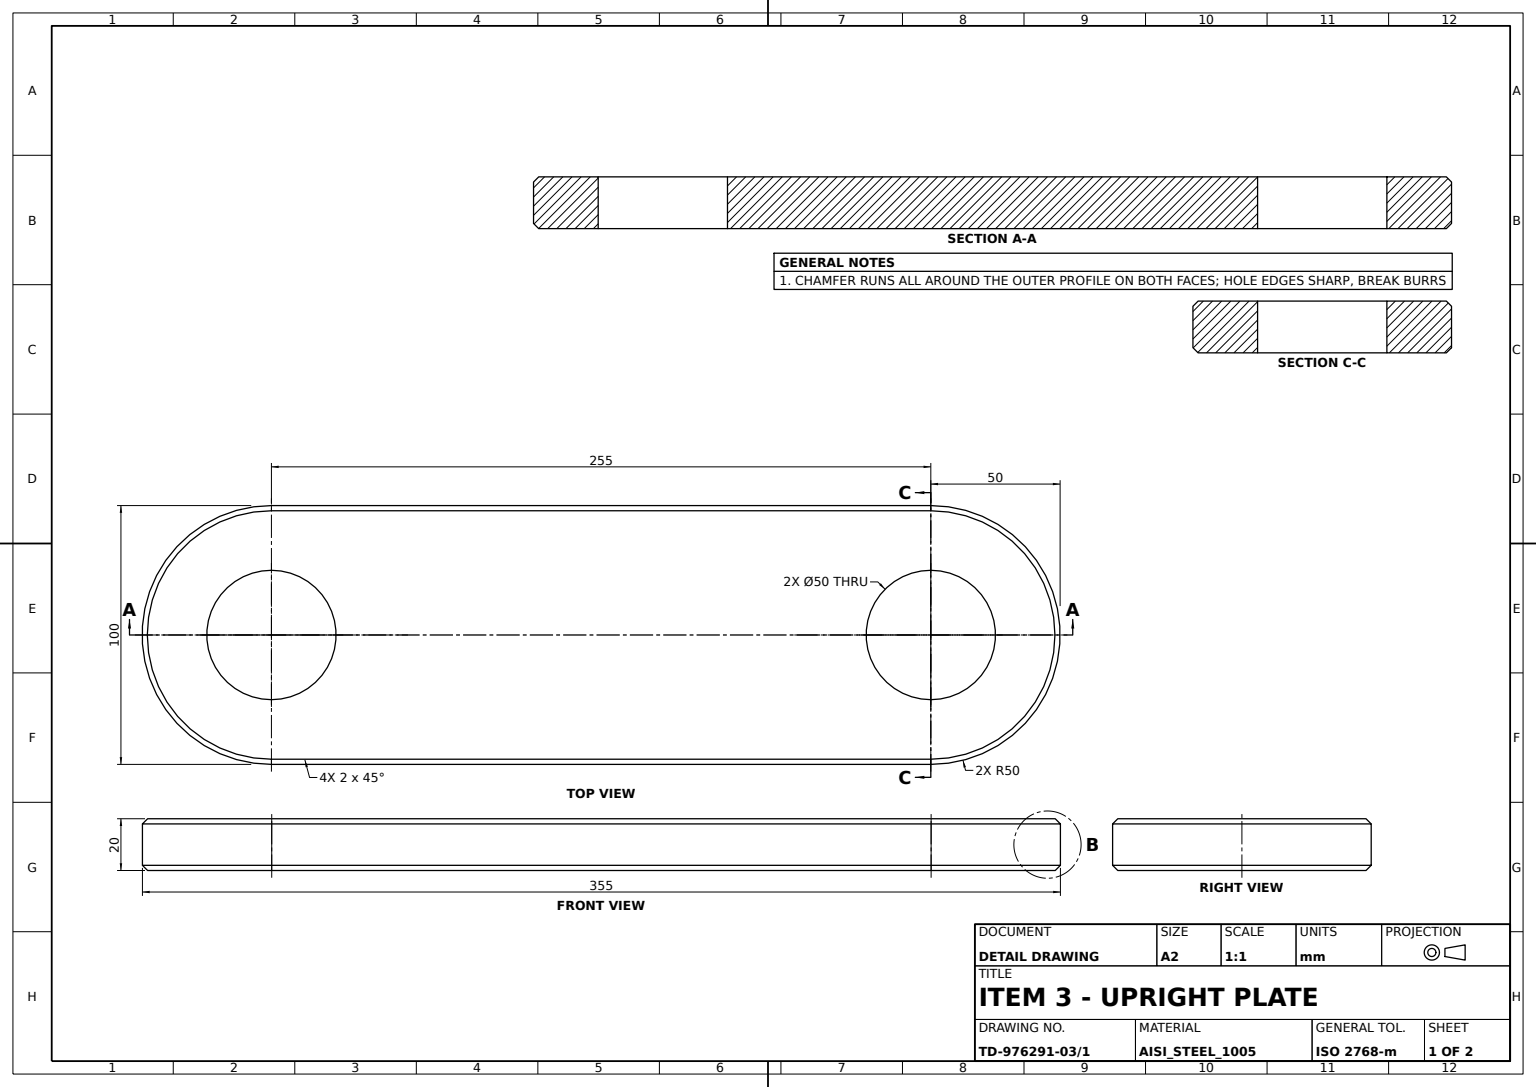
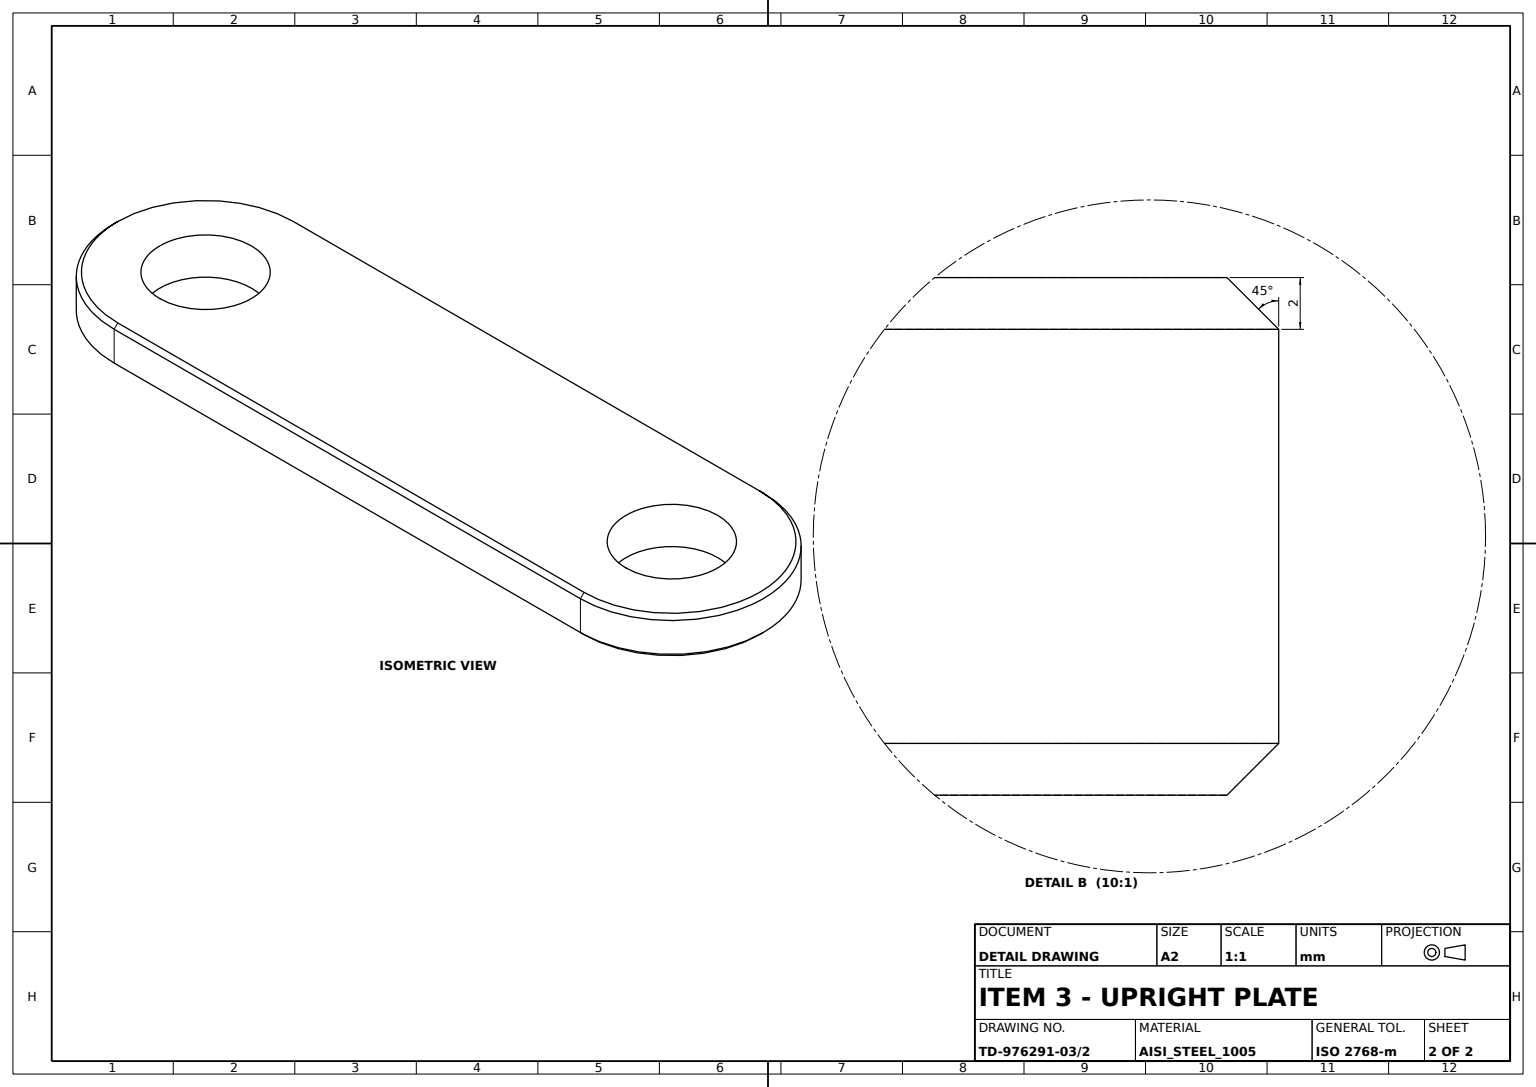
ISO-10303-21;
HEADER;
FILE_DESCRIPTION((''),'2;1');
FILE_NAME('','',(''),(''),'','','');
FILE_SCHEMA(('AUTOMOTIVE_DESIGN'));
ENDSEC;
DATA;
#1=APPLICATION_CONTEXT('');
#2=PRODUCT_CONTEXT('',#1,'mechanical');
#3=PRODUCT('','','',(#2));
#4=PRODUCT_DEFINITION_FORMATION('','',#3);
#5=PRODUCT_DEFINITION_CONTEXT('',#1,'design');
#6=PRODUCT_DEFINITION('','',#4,#5);
#7=PRODUCT_DEFINITION_SHAPE('','',#6);
#8=(LENGTH_UNIT()NAMED_UNIT(*)SI_UNIT(.MILLI.,.METRE.));
#9=(NAMED_UNIT(*)PLANE_ANGLE_UNIT()SI_UNIT($,.RADIAN.));
#10=(NAMED_UNIT(*)SI_UNIT($,.STERADIAN.)SOLID_ANGLE_UNIT());
#11=UNCERTAINTY_MEASURE_WITH_UNIT(LENGTH_MEASURE(0.005),#8,'distance_accuracy_value','');
#12=(GEOMETRIC_REPRESENTATION_CONTEXT(3)GLOBAL_UNCERTAINTY_ASSIGNED_CONTEXT((#11))GLOBAL_UNIT_ASSIGNED_CONTEXT((#8,#9,#10))REPRESENTATION_CONTEXT('',''));
#13=CARTESIAN_POINT('',(-50.,-2.,127.5));
#14=VERTEX_POINT('',#13);
#15=CARTESIAN_POINT('',(-48.,0.,127.5));
#16=VERTEX_POINT('',#15);
#17=DIRECTION('',(0.707106781,0.707106781,0.));
#18=VECTOR('',#17,1000.);
#19=LINE('',#13,#18);
#20=EDGE_CURVE('',#14,#16,#19,.T.);
#21=ORIENTED_EDGE('',*,*,#20,.F.);
#22=CARTESIAN_POINT('',(50.,-2.,127.5));
#23=VERTEX_POINT('',#22);
#24=CARTESIAN_POINT('',(0.,-2.,127.5));
#25=DIRECTION('',(0.,-1.,0.));
#26=DIRECTION('',(0.,0.,-1.));
#27=AXIS2_PLACEMENT_3D('',#24,#25,#26);
#28=CIRCLE('',#27,50.);
#29=EDGE_CURVE('',#23,#14,#28,.T.);
#30=ORIENTED_EDGE('',*,*,#29,.F.);
#31=CARTESIAN_POINT('',(48.,0.,127.5));
#32=VERTEX_POINT('',#31);
#33=DIRECTION('',(0.707106781,-0.707106781,0.));
#34=VECTOR('',#33,1000.);
#35=LINE('',#31,#34);
#36=EDGE_CURVE('',#32,#23,#35,.T.);
#37=ORIENTED_EDGE('',*,*,#36,.F.);
#38=CARTESIAN_POINT('',(0.,0.,127.5));
#39=AXIS2_PLACEMENT_3D('',#38,#25,#26);
#40=CIRCLE('',#39,48.);
#41=EDGE_CURVE('',#16,#32,#40,.F.);
#42=ORIENTED_EDGE('',*,*,#41,.F.);
#43=EDGE_LOOP('',(#21,#30,#37,#42));
#44=FACE_BOUND('',#43,.T.);
#45=CONICAL_SURFACE('',#27,50.,0.785398163);
#46=ADVANCED_FACE('',(#44),#45,.T.);
#47=CARTESIAN_POINT('',(50.,-18.,127.5));
#48=VERTEX_POINT('',#47);
#49=CARTESIAN_POINT('',(48.,-20.,127.5));
#50=VERTEX_POINT('',#49);
#51=DIRECTION('',(-0.707106781,-0.707106781,0.));
#52=VECTOR('',#51,1000.);
#53=LINE('',#47,#52);
#54=EDGE_CURVE('',#48,#50,#53,.T.);
#55=ORIENTED_EDGE('',*,*,#54,.F.);
#56=CARTESIAN_POINT('',(-50.,-18.,127.5));
#57=VERTEX_POINT('',#56);
#58=CARTESIAN_POINT('',(0.,-18.,127.5));
#59=AXIS2_PLACEMENT_3D('',#58,#25,#26);
#60=CIRCLE('',#59,50.);
#61=EDGE_CURVE('',#57,#48,#60,.F.);
#62=ORIENTED_EDGE('',*,*,#61,.F.);
#63=CARTESIAN_POINT('',(-48.,-20.,127.5));
#64=VERTEX_POINT('',#63);
#65=DIRECTION('',(-0.707106781,0.707106781,0.));
#66=VECTOR('',#65,1000.);
#67=LINE('',#63,#66);
#68=EDGE_CURVE('',#64,#57,#67,.T.);
#69=ORIENTED_EDGE('',*,*,#68,.F.);
#70=CARTESIAN_POINT('',(0.,-20.,127.5));
#71=AXIS2_PLACEMENT_3D('',#70,#25,#26);
#72=CIRCLE('',#71,48.);
#73=EDGE_CURVE('',#50,#64,#72,.T.);
#74=ORIENTED_EDGE('',*,*,#73,.F.);
#75=EDGE_LOOP('',(#55,#62,#69,#74));
#76=FACE_BOUND('',#75,.T.);
#77=DIRECTION('',(0.,1.,0.));
#78=DIRECTION('',(0.,0.,1.));
#79=AXIS2_PLACEMENT_3D('',#70,#77,#78);
#80=CONICAL_SURFACE('',#79,48.,0.785398163);
#81=ADVANCED_FACE('',(#76),#80,.T.);
#82=CARTESIAN_POINT('',(-50.,-20.,127.5));
#83=VECTOR('',#77,1000.);
#84=LINE('',#82,#83);
#85=EDGE_CURVE('',#57,#14,#84,.T.);
#86=ORIENTED_EDGE('',*,*,#85,.F.);
#87=ORIENTED_EDGE('',*,*,#61,.T.);
#88=CARTESIAN_POINT('',(50.,-20.,127.5));
#89=LINE('',#88,#83);
#90=EDGE_CURVE('',#48,#23,#89,.T.);
#91=ORIENTED_EDGE('',*,*,#90,.T.);
#92=ORIENTED_EDGE('',*,*,#29,.T.);
#93=EDGE_LOOP('',(#86,#87,#91,#92));
#94=FACE_BOUND('',#93,.T.);
#95=CYLINDRICAL_SURFACE('',#79,50.);
#96=ADVANCED_FACE('',(#94),#95,.T.);
#97=CARTESIAN_POINT('',(50.,-18.,-127.5));
#98=VERTEX_POINT('',#97);
#99=CARTESIAN_POINT('',(50.,-2.,-127.5));
#100=VERTEX_POINT('',#99);
#101=CARTESIAN_POINT('',(50.,-20.,-127.5));
#102=LINE('',#101,#83);
#103=EDGE_CURVE('',#98,#100,#102,.T.);
#104=ORIENTED_EDGE('',*,*,#103,.F.);
#105=CARTESIAN_POINT('',(-50.,-18.,-127.5));
#106=VERTEX_POINT('',#105);
#107=CARTESIAN_POINT('',(0.,-18.,-127.5));
#108=AXIS2_PLACEMENT_3D('',#107,#25,#26);
#109=CIRCLE('',#108,50.);
#110=EDGE_CURVE('',#98,#106,#109,.F.);
#111=ORIENTED_EDGE('',*,*,#110,.T.);
#112=CARTESIAN_POINT('',(-50.,-2.,-127.5));
#113=VERTEX_POINT('',#112);
#114=CARTESIAN_POINT('',(-50.,-20.,-127.5));
#115=LINE('',#114,#83);
#116=EDGE_CURVE('',#106,#113,#115,.T.);
#117=ORIENTED_EDGE('',*,*,#116,.T.);
#118=CARTESIAN_POINT('',(0.,-2.,-127.5));
#119=AXIS2_PLACEMENT_3D('',#118,#25,#26);
#120=CIRCLE('',#119,50.);
#121=EDGE_CURVE('',#113,#100,#120,.T.);
#122=ORIENTED_EDGE('',*,*,#121,.T.);
#123=EDGE_LOOP('',(#104,#111,#117,#122));
#124=FACE_BOUND('',#123,.T.);
#125=CARTESIAN_POINT('',(0.,-20.,-127.5));
#126=AXIS2_PLACEMENT_3D('',#125,#77,#78);
#127=CYLINDRICAL_SURFACE('',#126,50.);
#128=ADVANCED_FACE('',(#124),#127,.T.);
#129=VECTOR('',#26,1000.);
#130=LINE('',#13,#129);
#131=EDGE_CURVE('',#14,#113,#130,.T.);
#132=ORIENTED_EDGE('',*,*,#131,.T.);
#133=ORIENTED_EDGE('',*,*,#116,.F.);
#134=VECTOR('',#78,1000.);
#135=LINE('',#56,#134);
#136=EDGE_CURVE('',#106,#57,#135,.T.);
#137=ORIENTED_EDGE('',*,*,#136,.T.);
#138=ORIENTED_EDGE('',*,*,#85,.T.);
#139=EDGE_LOOP('',(#132,#133,#137,#138));
#140=FACE_BOUND('',#139,.T.);
#141=DIRECTION('',(1.,0.,0.));
#142=AXIS2_PLACEMENT_3D('',#82,#141,#26);
#143=PLANE('',#142);
#144=ADVANCED_FACE('',(#140),#143,.F.);
#145=CARTESIAN_POINT('',(25.,0.,127.5));
#146=VERTEX_POINT('',#145);
#147=AXIS2_PLACEMENT_3D('',#38,#25,#141);
#148=CIRCLE('',#147,25.);
#149=EDGE_CURVE('',#146,#146,#148,.T.);
#150=ORIENTED_EDGE('',*,*,#149,.F.);
#151=EDGE_LOOP('',(#150));
#152=FACE_BOUND('',#151,.T.);
#153=CARTESIAN_POINT('',(25.,-20.,127.5));
#154=VERTEX_POINT('',#153);
#155=AXIS2_PLACEMENT_3D('',#70,#25,#141);
#156=CIRCLE('',#155,25.);
#157=EDGE_CURVE('',#154,#154,#156,.T.);
#158=ORIENTED_EDGE('',*,*,#157,.T.);
#159=EDGE_LOOP('',(#158));
#160=FACE_BOUND('',#159,.T.);
#161=CYLINDRICAL_SURFACE('',#79,25.);
#162=ADVANCED_FACE('',(#152,#160),#161,.F.);
#163=CARTESIAN_POINT('',(25.,-20.,-127.5));
#164=VERTEX_POINT('',#163);
#165=AXIS2_PLACEMENT_3D('',#125,#25,#141);
#166=CIRCLE('',#165,25.);
#167=EDGE_CURVE('',#164,#164,#166,.T.);
#168=ORIENTED_EDGE('',*,*,#167,.F.);
#169=EDGE_LOOP('',(#168));
#170=FACE_BOUND('',#169,.T.);
#171=CARTESIAN_POINT('',(-48.,-20.,-127.5));
#172=VERTEX_POINT('',#171);
#173=CARTESIAN_POINT('',(48.,-20.,-127.5));
#174=VERTEX_POINT('',#173);
#175=AXIS2_PLACEMENT_3D('',#125,#25,#26);
#176=CIRCLE('',#175,48.);
#177=EDGE_CURVE('',#172,#174,#176,.T.);
#178=ORIENTED_EDGE('',*,*,#177,.T.);
#179=LINE('',#49,#134);
#180=EDGE_CURVE('',#174,#50,#179,.T.);
#181=ORIENTED_EDGE('',*,*,#180,.T.);
#182=ORIENTED_EDGE('',*,*,#73,.T.);
#183=LINE('',#171,#129);
#184=EDGE_CURVE('',#64,#172,#183,.T.);
#185=ORIENTED_EDGE('',*,*,#184,.T.);
#186=EDGE_LOOP('',(#178,#181,#182,#185));
#187=FACE_BOUND('',#186,.T.);
#188=ORIENTED_EDGE('',*,*,#157,.F.);
#189=EDGE_LOOP('',(#188));
#190=FACE_BOUND('',#189,.T.);
#191=PLANE('',#175);
#192=ADVANCED_FACE('',(#170,#187,#190),#191,.T.);
#193=CARTESIAN_POINT('',(48.,0.,-127.5));
#194=VERTEX_POINT('',#193);
#195=LINE('',#193,#34);
#196=EDGE_CURVE('',#194,#100,#195,.T.);
#197=ORIENTED_EDGE('',*,*,#196,.F.);
#198=LINE('',#193,#129);
#199=EDGE_CURVE('',#32,#194,#198,.T.);
#200=ORIENTED_EDGE('',*,*,#199,.F.);
#201=ORIENTED_EDGE('',*,*,#36,.T.);
#202=LINE('',#99,#134);
#203=EDGE_CURVE('',#100,#23,#202,.T.);
#204=ORIENTED_EDGE('',*,*,#203,.F.);
#205=EDGE_LOOP('',(#197,#200,#201,#204));
#206=FACE_BOUND('',#205,.T.);
#207=AXIS2_PLACEMENT_3D('',#99,#51,#78);
#208=PLANE('',#207);
#209=ADVANCED_FACE('',(#206),#208,.F.);
#210=ORIENTED_EDGE('',*,*,#121,.F.);
#211=CARTESIAN_POINT('',(-48.,0.,-127.5));
#212=VERTEX_POINT('',#211);
#213=LINE('',#112,#18);
#214=EDGE_CURVE('',#113,#212,#213,.T.);
#215=ORIENTED_EDGE('',*,*,#214,.T.);
#216=CARTESIAN_POINT('',(0.,0.,-127.5));
#217=AXIS2_PLACEMENT_3D('',#216,#25,#26);
#218=CIRCLE('',#217,48.);
#219=EDGE_CURVE('',#194,#212,#218,.F.);
#220=ORIENTED_EDGE('',*,*,#219,.F.);
#221=ORIENTED_EDGE('',*,*,#196,.T.);
#222=EDGE_LOOP('',(#210,#215,#220,#221));
#223=FACE_BOUND('',#222,.T.);
#224=CONICAL_SURFACE('',#119,50.,0.785398163);
#225=ADVANCED_FACE('',(#223),#224,.T.);
#226=ORIENTED_EDGE('',*,*,#54,.T.);
#227=ORIENTED_EDGE('',*,*,#180,.F.);
#228=LINE('',#97,#52);
#229=EDGE_CURVE('',#98,#174,#228,.T.);
#230=ORIENTED_EDGE('',*,*,#229,.F.);
#231=LINE('',#97,#129);
#232=EDGE_CURVE('',#48,#98,#231,.T.);
#233=ORIENTED_EDGE('',*,*,#232,.F.);
#234=EDGE_LOOP('',(#226,#227,#230,#233));
#235=FACE_BOUND('',#234,.T.);
#236=AXIS2_PLACEMENT_3D('',#173,#33,#26);
#237=PLANE('',#236);
#238=ADVANCED_FACE('',(#235),#237,.T.);
#239=CARTESIAN_POINT('',(25.,0.,-127.5));
#240=VERTEX_POINT('',#239);
#241=AXIS2_PLACEMENT_3D('',#216,#25,#141);
#242=CIRCLE('',#241,25.);
#243=EDGE_CURVE('',#240,#240,#242,.T.);
#244=ORIENTED_EDGE('',*,*,#243,.F.);
#245=EDGE_LOOP('',(#244));
#246=FACE_BOUND('',#245,.T.);
#247=ORIENTED_EDGE('',*,*,#167,.T.);
#248=EDGE_LOOP('',(#247));
#249=FACE_BOUND('',#248,.T.);
#250=CYLINDRICAL_SURFACE('',#126,25.);
#251=ADVANCED_FACE('',(#246,#249),#250,.F.);
#252=ORIENTED_EDGE('',*,*,#232,.T.);
#253=ORIENTED_EDGE('',*,*,#103,.T.);
#254=ORIENTED_EDGE('',*,*,#203,.T.);
#255=ORIENTED_EDGE('',*,*,#90,.F.);
#256=EDGE_LOOP('',(#252,#253,#254,#255));
#257=FACE_BOUND('',#256,.T.);
#258=DIRECTION('',(-1.,0.,0.));
#259=AXIS2_PLACEMENT_3D('',#101,#258,#78);
#260=PLANE('',#259);
#261=ADVANCED_FACE('',(#257),#260,.F.);
#262=ORIENTED_EDGE('',*,*,#177,.F.);
#263=LINE('',#171,#66);
#264=EDGE_CURVE('',#172,#106,#263,.T.);
#265=ORIENTED_EDGE('',*,*,#264,.T.);
#266=ORIENTED_EDGE('',*,*,#110,.F.);
#267=ORIENTED_EDGE('',*,*,#229,.T.);
#268=EDGE_LOOP('',(#262,#265,#266,#267));
#269=FACE_BOUND('',#268,.T.);
#270=CONICAL_SURFACE('',#126,48.,0.785398163);
#271=ADVANCED_FACE('',(#269),#270,.T.);
#272=LINE('',#211,#134);
#273=EDGE_CURVE('',#212,#16,#272,.T.);
#274=ORIENTED_EDGE('',*,*,#273,.F.);
#275=ORIENTED_EDGE('',*,*,#214,.F.);
#276=ORIENTED_EDGE('',*,*,#131,.F.);
#277=ORIENTED_EDGE('',*,*,#20,.T.);
#278=EDGE_LOOP('',(#274,#275,#276,#277));
#279=FACE_BOUND('',#278,.T.);
#280=AXIS2_PLACEMENT_3D('',#13,#33,#26);
#281=PLANE('',#280);
#282=ADVANCED_FACE('',(#279),#281,.F.);
#283=ORIENTED_EDGE('',*,*,#243,.T.);
#284=EDGE_LOOP('',(#283));
#285=FACE_BOUND('',#284,.T.);
#286=ORIENTED_EDGE('',*,*,#149,.T.);
#287=EDGE_LOOP('',(#286));
#288=FACE_BOUND('',#287,.T.);
#289=ORIENTED_EDGE('',*,*,#219,.T.);
#290=ORIENTED_EDGE('',*,*,#273,.T.);
#291=ORIENTED_EDGE('',*,*,#41,.T.);
#292=ORIENTED_EDGE('',*,*,#199,.T.);
#293=EDGE_LOOP('',(#289,#290,#291,#292));
#294=FACE_BOUND('',#293,.T.);
#295=PLANE('',#217);
#296=ADVANCED_FACE('',(#285,#288,#294),#295,.F.);
#297=ORIENTED_EDGE('',*,*,#184,.F.);
#298=ORIENTED_EDGE('',*,*,#68,.T.);
#299=ORIENTED_EDGE('',*,*,#136,.F.);
#300=ORIENTED_EDGE('',*,*,#264,.F.);
#301=EDGE_LOOP('',(#297,#298,#299,#300));
#302=FACE_BOUND('',#301,.T.);
#303=AXIS2_PLACEMENT_3D('',#171,#51,#78);
#304=PLANE('',#303);
#305=ADVANCED_FACE('',(#302),#304,.T.);
#306=CLOSED_SHELL('',(#46,#81,#96,#128,#144,#162,#192,#209,#225,#238,#251,#261,#271,#282,#296,#305));
#307=MANIFOLD_SOLID_BREP('',#306);
#308=ADVANCED_BREP_SHAPE_REPRESENTATION('',(#307),#12);
#309=SHAPE_DEFINITION_REPRESENTATION(#7,#308);
ENDSEC;
END-ISO-10303-21;
